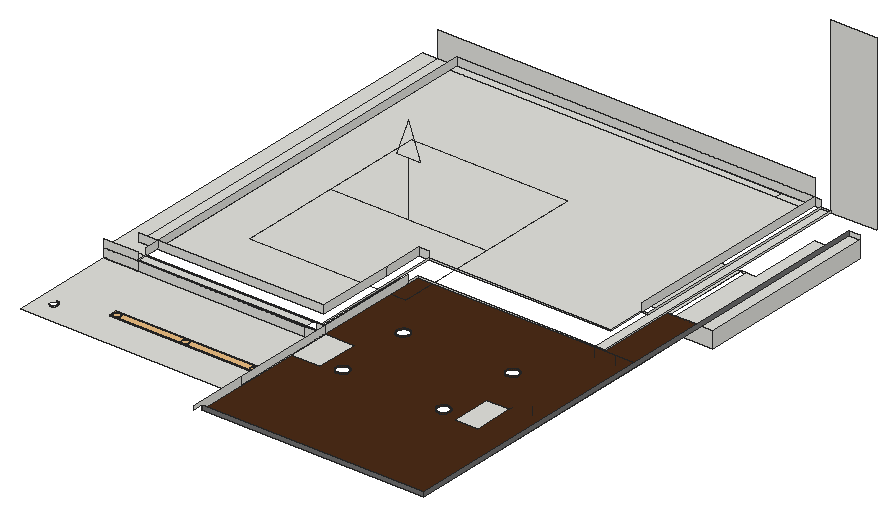
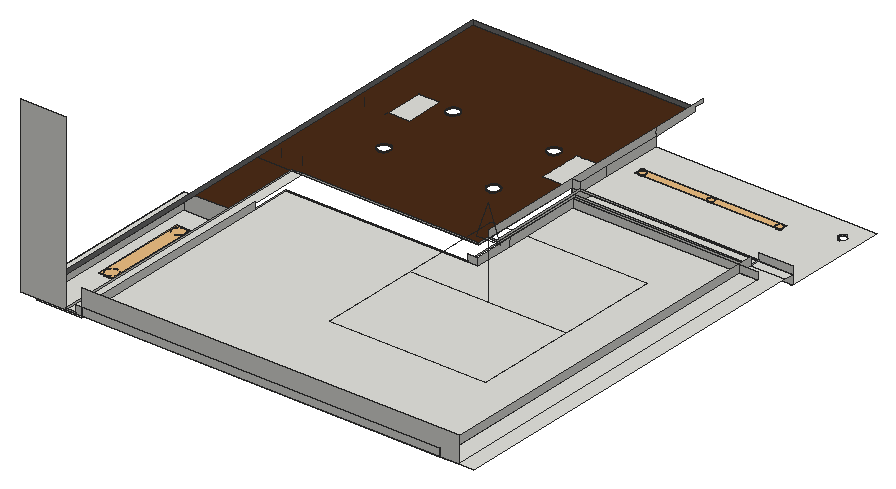
# SketchUp Ruby script. Lengths in inches.
U = 1.inch
M = Sketchup.active_model
def pt(a) = Geom::Point3d.new(a.map { |v| v * U })
def face(e, loops, mat)
  f = e.add_face(loops[0].map { |a| pt(a) })
  loops[1..].each { |l| e.add_face(l.map { |a| pt(a) }).erase! }
  f.material = f.back_material = mat if mat
  f
end
# faces: each face lists its corners as indices into pts; further lists are holes
def faces(e, pts, list, mat = nil) = list.each { |f| face(e, (f[0].is_a?(Array) ? f : [f]).map { |l| l.map { |i| pts[i] } }, mat) }
# xy, xz, yz: faces in a plane at the given z, y or x. An outline is a flat list of corners, or four numbers for a rectangle; further outlines are holes
def ring(l) = l.size == 4 ? [[l[0], l[1]], [l[2], l[1]], [l[2], l[3]], [l[0], l[3]]] : l.each_slice(2).to_a
def flat(e, list, mat, &to3) = list.each { |f| face(e, (f[0].is_a?(Array) ? f : [f]).map { |l| ring(l).map { |u, v| to3.(u, v) } }, mat) }
def xy(e, z, list, mat = nil) = flat(e, list, mat) { |x, y| [x, y, z] }
def xz(e, y, list, mat = nil) = flat(e, list, mat) { |x, z| [x, y, z] }
def yz(e, x, list, mat = nil) = flat(e, list, mat) { |y, z| [x, y, z] }
def lines(e, pts, list) = list.each { |a, b| e.add_line(pt(pts[a]), pt(pts[b])) }
# prism: a flat outline (further loops are holes) pulled along v
def prism(e, loops, v, mat = nil)
  f = face(e, loops, mat); d = Geom::Vector3d.new(v.map { |x| x * U })
  f.pushpull(f.normal.samedirection?(d) ? d.length : -d.length)
end
def box(e, o, s, mat = nil) = prism(e, [[o, [o[0] + s[0], o[1], o[2]], [o[0] + s[0], o[1] + s[1], o[2]], [o[0], o[1] + s[1], o[2]]]], [0, 0, s[2]], mat)
def at(x, y, z, deg = 0) = Geom::Transformation.translation(pt([x, y, z])) * Geom::Transformation.rotation(ORIGIN, Z_AXIS, deg.degrees)
def axes(o, x, y, z) = Geom::Transformation.new([*x, 0, *y, 0, *z, 0, *pt(o).to_a, 1])
def part(name) = M.definitions.add(name)
# library, detail: a bought-in or finely detailed component or shape, given as its bounding box
def library(name, o, s) = part(name).tap { |d| box(d.entities, o, s) }
def detail(e, o, s) = box(e.add_group.entities, o, s)
def put(e, d, t, mat = nil) = e.add_instance(d, t).tap { |i| i.material = mat if mat }
def group(e, t, mat = nil) = e.add_group.tap { |g| g.transformation = t; g.material = mat if mat }.entities
root = M.entities
M.materials.add("[Color M05]").color = [114, 114, 114]
M.materials.add("[Wood Veneer 01]").color = [76, 44, 23]
c1 = library("Group\#20",[-0.5,-0.5,-0.1],[139.5,7.875,0.2])
c2 = part("Group266\#1")
p = [[0,0,0],[0,0,-53.16],[-11.52,0,-53.16],[75.01,-97.09,0],[-75.01,-97.09,0],[75.01,97.09,0],
  [75.01,0,0],[-75.01,97.09,0],[11.52,0,-53.16],[-75.01,0,0],[0,0,-86.05]]
lines(c2.entities,p,[[0,1],[1,2],[3,4],[5,6],[7,5],[1,8],[9,0],[0,6],[8,10],[4,9],[6,3],[2,10],
  [9,7]])
c3 = part("Rectangle Light\#1")
put(c3.entities,c2,at(0,0,0))
c4 = library("Group\#22",[-0.5,-0.5,-0.1],[13.19,93.55,0.2])
xy(root,102.625,[[[3349.13,1821.9,3349.13,1844.2,3339.91,1844.2,3339.91,1928.83,3349.13,1928.83,3349.13,1998.71,3392.88,1998.71,3392.88,1821.9],[3374.07,1926.22,3375.65,1926.42,3377.12,1927.03,3378.38,1928,3379.35,1929.26,3379.96,1930.73,3380.16,1932.31,3379.96,1933.89,3379.35,1935.35,3378.38,1936.62,3377.12,1937.58,3375.65,1938.19,3374.07,1938.4,3372.49,1938.19,3371.02,1937.58,3369.76,1936.62,3368.79,1935.35,3368.1875,1933.89,3367.98,1932.31,3368.1875,1930.73,3368.79,1929.26,3369.76,1928,3371.02,1927.03,3372.49,1926.42],[3374.07,1845.85,3375.625,1846.05,3377.07,1846.65,3378.3125,1847.61,3379.27,1848.85,3379.87,1850.3,3380.07,1851.85,3379.87,1853.4,3379.27,1854.85,3378.3125,1856.09,3377.07,1857.05,3375.625,1857.65,3374.07,1857.85,3372.52,1857.65,3371.07,1857.05,3369.83,1856.09,3368.875,1854.85,3368.28,1853.4,3368.07,1851.85,3368.28,1850.3,3368.875,1848.85,3369.83,1847.61,3371.07,1846.65,3372.52,1846.05]],[3240.94,1844.2,3334.66,1928.14],[3334.66,1844.2,3335.34,1928.83],[3240.94,1928.14,3334.66,1928.83],[3335.34,1928.14,3336.03,1928.14,3336.03,1928.27,3339.91,1928.27,3339.91,1928.83,3335.34,1928.83],
  [3336.03,1928.14,3339.91,1928.27]])
xy(root,109.625,[[[2957.51,1535.54,3169.48,1636.04],[2972.07,1553.19,2973.125,1553.33,2974.1,1553.73,2974.95,1554.38,2975.59,1555.22,2976,1556.2,2976.14,1557.25,2976,1558.3,2975.59,1559.28,2974.95,1560.125,2974.1,1560.77,2973.125,1561.18,2972.07,1561.31,2971.02,1561.18,2970.04,1560.77,2969.2,1560.125,2968.55,1559.28,2968.15,1558.3,2968.01,1557.25,2968.15,1556.2,2968.55,1555.22,2969.2,1554.38,2970.04,1553.73,2971.02,1553.33],[3020.13,1569.87,3021.02,1569.99,3021.85,1570.33,3022.56,1570.875,3023.11,1571.59,3023.45,1572.42,3023.57,1573.31,3023.45,1574.2,3023.11,1575.02,3022.56,1575.74,3021.85,1576.28,3021.02,1576.625,3020.13,1576.74,3019.24,1576.625,3018.41,1576.28,3017.7,1575.74,3017.15,1575.02,3016.81,1574.2,3016.69,1573.31,3016.81,1572.42,3017.15,1571.59,3017.7,1570.875,3018.41,1570.33,3019.24,1569.99],[3085.94,1569.87,3086.83,1569.99,3087.66,1570.33,3088.37,1570.875,3088.92,1571.59,3089.26,1572.42,3089.38,1573.31,3089.26,1574.2,3088.92,1575.02,3088.37,1575.74,3087.66,1576.28,3086.83,1576.625,3085.94,1576.74,3085.05,1576.625,3084.22,1576.28,3083.51,1575.74,3082.96,1575.02,3082.62,1574.2,3082.5,1573.31,3082.62,1572.42,3082.96,1571.59,3083.51,1570.875,3084.22,1570.33,3085.05,1569.99],[3151.75,1569.87,3152.64,1569.99,3153.47,1570.33,3154.19,1570.875,3154.73,1571.59,3155.07,1572.42,3155.19,1573.31,3155.07,1574.2,3154.73,1575.02,3154.19,1575.74,3153.47,1576.28,3152.64,1576.625,3151.75,1576.74,3150.86,1576.625,3150.04,1576.28,3149.32,1575.74,3148.78,1575.02,3148.43,1574.2,3148.32,1573.31,3148.43,1572.42,3148.78,1571.59,3149.32,1570.875,3150.04,1570.33,3150.86,1569.99]]])
xy(root,118.5,[[3169.48,1595.04,3196.91,1635.98],[3327.63,1595.04,3349.13,1632.6],[2957.51,1636.04,2989.82,1645.27],[2989.82,1636.04,3150.65,1645.27],[2957.51,1645.27,2989.82,1645.27,2989.82,1659.57,2972.24,1659.57,2972.24,2018.36,2957.51,2018.36],
  [2972.24,1659.57,2989.82,2018.36],[2989.82,1659.57,2989.82,2010.98,3333.43,2010.98,3333.43,1773.67,3149.44,1773.67,3149.44,1659.57],[3339.91,1746.92,3349.13,2018.36],[3382.57,1821.9,3392.88,1998.71],[2989.82,2010.98,3302.57,2018.36],
  [3302.57,2010.98,3333.43,2018.36]])
xy(root,118.5,[[[3169.48,1488.17,3169.48,1595.04,3196.91,1595.04,3196.91,1635.98,3169.48,1635.98,3169.48,1746.92,3382.57,1746.92,3382.57,1488.17],[3327.63,1595.04,3349.13,1632.6],[3311.11,1595.24,3312.66,1595.44,3314.11,1596.04,3315.35,1596.99,3316.31,1598.24,3316.91,1599.68,3317.11,1601.24,3316.91,1602.79,3316.31,1604.24,3315.35,1605.48,3314.11,1606.43,3312.66,1607.03,3311.11,1607.24,3309.56,1607.03,3308.11,1606.43,3306.87,1605.48,3305.92,1604.24,3305.32,1602.79,3305.11,1601.24,3305.32,1599.68,3305.92,1598.24,3306.87,1596.99,3308.11,1596.04,3309.56,1595.44],[3214.3,1595.24,3215.85,1595.44,3217.3,1596.04,3218.54,1596.99,3219.5,1598.24,3220.09,1599.68,3220.3,1601.24,3220.09,1602.79,3219.5,1604.24,3218.54,1605.48,3217.3,1606.43,3215.85,1607.03,3214.3,1607.24,3212.75,1607.03,3211.3,1606.43,3210.06,1605.48,3209.1,1604.24,3208.5,1602.79,3208.3,1601.24,3208.5,1599.68,3209.1,1598.24,3210.06,1596.99,3211.3,1596.04,3212.75,1595.44],[3214.3,1667.99,3215.85,1668.19,3217.3,1668.79,3218.54,1669.74,3219.5,1670.99,3220.09,1672.43,3220.3,1673.99,3220.09,1675.54,3219.5,1676.99,3218.54,1678.23,3217.3,1679.18,3215.85,1679.78,3214.3,1679.99,3212.75,1679.78,3211.3,1679.18,3210.06,1678.23,3209.1,1676.99,3208.5,1675.54,3208.3,1673.99,3208.5,1672.43,3209.1,1670.99,3210.06,1669.74,3211.3,1668.79,3212.75,1668.19],[3316.66,1671.22,3318.21,1671.43,3319.66,1672.03,3320.9,1672.98,3321.86,1674.22,3322.46,1675.67,3322.66,1677.22,3322.46,1678.77,3321.86,1680.22,3320.9,1681.46,3319.66,1682.42,3318.21,1683.02,3316.66,1683.22,3315.11,1683.02,3313.66,1682.42,3312.42,1681.46,3311.46,1680.22,3310.87,1678.77,3310.66,1677.22,3310.87,1675.67,3311.46,1674.22,3312.42,1672.98,3313.66,1672.03,3315.11,1671.43]],[3349.13,1746.92,3382.57,1821.9]],"[Wood Veneer 01]")
xz(root,1488.17,[[3169.48,118.5,3382.57,122.875]],"[Color M05]")
xz(root,1636.04,[[2957.51,109.5,2989.82,109.625],[2957.51,109.625,2989.82,118.5],[2989.82,109.625,3150.65,118.5],[3150.65,109.625,3169.48,118.5],[2957.51,118.5,2989.82,126],
  [2989.82,118.5,3162.07,119.75],[3162.07,118.5,3169.48,126]])
xz(root,1645.27,[[2989.82,118.5,3159.13,119.75]])
xz(root,1659.57,[[2972.24,118.5,3149.44,126]])
xz(root,1735.1,[[3162.07,118.5,3169.48,119.75]])
xz(root,1746.92,[[3169.48,118.5,3339.91,119.75],[3339.91,118.5,3349.13,119.75]])
xz(root,1773.67,[[3149.44,118.5,3159.13,126],[3159.13,118.5,3333.43,119.75]])
xz(root,1810.9,[[3333.43,118.5,3339.91,119.75]])
xz(root,1821.9,[[3349.13,102.625,3392.88,118.5]])
xz(root,1998.71,[[3382.57,118.5,3392.88,122.875]])
xz(root,2018.36,[[2972.24,118.5,2972.24,142.875,3333.43,142.875,3333.43,126,2989.82,126,2989.82,118.5],[2989.82,118.5,3333.43,126],[3333.43,118.5,3339.91,126],[3339.91,118.5,3349.13,119.75],[3349.13,118.5,3392.88,283.9375]])
yz(root,2989.82,[[1636.04,118.5,1645.27,119.75],[1645.27,118.5,2018.36,126]])
yz(root,3149.44,[[1659.57,118.5,1735.1,126],[1735.1,118.5,1773.67,126]])
yz(root,3159.13,[[1645.27,118.5,1773.67,119.75]])
yz(root,3162.07,[[1636.04,118.5,1735.1,119.75]])
yz(root,3169.48,[[1535.54,109.625,1595.04,118.5],[1595.04,109.625,1635.98,118.5],[1635.98,109.625,1636.04,118.5],[1488.17,118.5,1488.17,122.875,1478.85,122.875,1478.85,126,1535.54,126,1535.54,118.5],[1535.54,118.5,1636.04,126],
  [1636.04,118.5,1735.1,126],[1735.1,118.5,1746.92,119.75]])
yz(root,3333.43,[[1773.67,118.5,1810.9,119.75],[1810.9,118.5,2018.36,126]])
yz(root,3339.91,[[1810.9,118.5,2018.36,119.75]])
yz(root,3349.13,[[1746.92,118.5,2018.36,119.75]])
yz(root,3382.57,[[1488.17,118.5,1998.71,122.875]],"[Color M05]")
yz(root,3392.88,[[1821.9,102.625,1998.71,118.5]])
p = [[3374.07,1845.85,102.625],[3372.52,1846.05,102.625],[3372.52,1846.05,103.9375],[3374.07,1845.85,103.9375],[3375.625,1846.05,102.625],[3375.625,1846.05,103.9375],
  [3371.07,1846.65,102.625],[3371.07,1846.65,103.9375],[3377.07,1846.65,102.625],[3377.07,1846.65,103.9375],[3369.83,1847.61,102.625],[3369.83,1847.61,103.9375],
  [3378.3125,1847.61,102.625],[3378.3125,1847.61,103.9375],[3368.875,1848.85,102.625],[3368.875,1848.85,103.9375],[3379.27,1848.85,102.625],[3379.27,1848.85,103.9375],
  [3368.28,1850.3,102.625],[3368.28,1850.3,103.9375],[3379.87,1850.3,102.625],[3379.87,1850.3,103.9375],[3368.07,1851.85,102.625],[3368.07,1851.85,103.9375],
  [3380.07,1851.85,102.625],[3380.07,1851.85,103.9375],[3368.28,1853.4,102.625],[3368.28,1853.4,103.9375],[3379.87,1853.4,102.625],[3379.87,1853.4,103.9375],
  [3368.875,1854.85,102.625],[3368.875,1854.85,103.9375],[3379.27,1854.85,102.625],[3379.27,1854.85,103.9375],[3369.83,1856.09,102.625],[3369.83,1856.09,103.9375],
  [3378.3125,1856.09,102.625],[3378.3125,1856.09,103.9375],[3371.07,1857.05,102.625],[3371.07,1857.05,103.9375],[3377.07,1857.05,102.625],[3377.07,1857.05,103.9375],
  [3372.52,1857.65,102.625],[3372.52,1857.65,103.9375],[3375.625,1857.65,102.625],[3375.625,1857.65,103.9375],[3374.07,1857.85,102.625],[3374.07,1857.85,103.9375],
  [3374.07,1926.22,102.625],[3372.49,1926.42,102.625],[3372.49,1926.42,103.9375],[3374.07,1926.22,103.9375],[3375.65,1926.42,102.625],[3375.65,1926.42,103.9375],
  [3371.02,1927.03,102.625],[3371.02,1927.03,103.9375],[3377.12,1927.03,102.625],[3377.12,1927.03,103.9375],[3369.76,1928,102.625],[3369.76,1928,103.9375],
  [3378.38,1928,102.625],[3378.38,1928,103.9375],[3368.79,1929.26,102.625],[3368.79,1929.26,103.9375],[3379.35,1929.26,102.625],[3379.35,1929.26,103.9375],
  [3368.1875,1930.73,102.625],[3368.1875,1930.73,103.9375],[3379.96,1930.73,102.625],[3379.96,1930.73,103.9375],[3367.98,1932.31,102.625],[3367.98,1932.31,103.9375],
  [3380.16,1932.31,102.625],[3380.16,1932.31,103.9375],[3368.1875,1933.89,102.625],[3368.1875,1933.89,103.9375],[3379.96,1933.89,102.625],[3379.96,1933.89,103.9375],
  [3368.79,1935.35,102.625],[3368.79,1935.35,103.9375],[3379.35,1935.35,102.625],[3379.35,1935.35,103.9375],[3369.76,1936.62,102.625],[3369.76,1936.62,103.9375],
  [3378.38,1936.62,102.625],[3378.38,1936.62,103.9375],[3371.02,1937.58,102.625],[3371.02,1937.58,103.9375],[3377.12,1937.58,102.625],[3377.12,1937.58,103.9375],
  [3372.49,1938.19,102.625],[3372.49,1938.19,103.9375],[3375.65,1938.19,102.625],[3375.65,1938.19,103.9375],[3374.07,1938.4,102.625],[3374.07,1938.4,103.9375],
  [2973.125,1553.33,109.625],[2972.07,1553.19,109.625],[2972.07,1553.19,110.5625],[2973.125,1553.33,110.5625],[2974.1,1553.73,109.625],[2974.1,1553.73,110.5625],
  [2974.95,1554.38,109.625],[2974.95,1554.38,110.5625],[2975.59,1555.22,109.625],[2975.59,1555.22,110.5625],[2976,1556.2,109.625],[2976,1556.2,110.5625],
  [2976.14,1557.25,109.625],[2976.14,1557.25,110.5625],[2976,1558.3,109.625],[2976,1558.3,110.5625],[2975.59,1559.28,109.625],[2975.59,1559.28,110.5625],
  [2974.95,1560.125,109.625],[2974.95,1560.125,110.5625],[2974.1,1560.77,109.625],[2974.1,1560.77,110.5625],[2973.125,1561.18,109.625],[2973.125,1561.18,110.5625],
  [2972.07,1561.31,109.625],[2972.07,1561.31,110.5625],[3020.13,1569.87,109.625],[3019.24,1569.99,109.625],[3019.24,1569.99,110.0625],[3020.13,1569.87,110.0625],
  [3021.02,1569.99,109.625],[3021.02,1569.99,110.0625],[3085.94,1569.87,109.625],[3085.05,1569.99,109.625],[3085.05,1569.99,110.0625],[3085.94,1569.87,110.0625],
  [3086.83,1569.99,109.625],[3086.83,1569.99,110.0625],[3151.75,1569.87,109.625],[3150.86,1569.99,109.625],[3150.86,1569.99,110.0625],[3151.75,1569.87,110.0625],
  [3152.64,1569.99,109.625],[3152.64,1569.99,110.0625],[3018.41,1570.33,109.625],[3018.41,1570.33,110.0625],[3021.85,1570.33,109.625],[3021.85,1570.33,110.0625],
  [3084.22,1570.33,109.625],[3084.22,1570.33,110.0625],[3087.66,1570.33,109.625],[3087.66,1570.33,110.0625],[3150.04,1570.33,109.625],[3150.04,1570.33,110.0625],
  [3153.47,1570.33,109.625],[3153.47,1570.33,110.0625],[3017.7,1570.875,109.625],[3017.7,1570.875,110.0625],[3022.56,1570.875,109.625],[3022.56,1570.875,110.0625],
  [3083.51,1570.875,109.625],[3083.51,1570.875,110.0625],[3088.37,1570.875,109.625],[3088.37,1570.875,110.0625],[3149.32,1570.875,109.625],[3149.32,1570.875,110.0625],
  [3154.19,1570.875,109.625],[3154.19,1570.875,110.0625],[3017.15,1571.59,109.625],[3017.15,1571.59,110.0625],[3023.11,1571.59,109.625],[3023.11,1571.59,110.0625],
  [3082.96,1571.59,109.625],[3082.96,1571.59,110.0625],[3088.92,1571.59,109.625],[3088.92,1571.59,110.0625],[3148.78,1571.59,109.625],[3148.78,1571.59,110.0625],
  [3154.73,1571.59,109.625],[3154.73,1571.59,110.0625],[3016.81,1572.42,109.625],[3016.81,1572.42,110.0625],[3023.45,1572.42,109.625],[3023.45,1572.42,110.0625],
  [3082.62,1572.42,109.625],[3082.62,1572.42,110.0625],[3089.26,1572.42,109.625],[3089.26,1572.42,110.0625],[3148.43,1572.42,109.625],[3148.43,1572.42,110.0625],
  [3155.07,1572.42,109.625],[3155.07,1572.42,110.0625],[3016.69,1573.31,109.625],[3016.69,1573.31,110.0625],[3023.57,1573.31,109.625],[3023.57,1573.31,110.0625],
  [3082.5,1573.31,109.625],[3082.5,1573.31,110.0625],[3089.38,1573.31,109.625],[3089.38,1573.31,110.0625],[3148.32,1573.31,109.625],[3148.32,1573.31,110.0625],
  [3155.19,1573.31,109.625],[3155.19,1573.31,110.0625],[3016.81,1574.2,109.625],[3016.81,1574.2,110.0625],[3023.45,1574.2,109.625],[3023.45,1574.2,110.0625],
  [3082.62,1574.2,109.625],[3082.62,1574.2,110.0625],[3089.26,1574.2,109.625],[3089.26,1574.2,110.0625],[3148.43,1574.2,109.625],[3148.43,1574.2,110.0625],
  [3155.07,1574.2,109.625],[3155.07,1574.2,110.0625],[3017.15,1575.02,109.625],[3017.15,1575.02,110.0625],[3023.11,1575.02,109.625],[3023.11,1575.02,110.0625],
  [3082.96,1575.02,109.625],[3082.96,1575.02,110.0625],[3088.92,1575.02,109.625],[3088.92,1575.02,110.0625],[3148.78,1575.02,109.625],[3148.78,1575.02,110.0625],
  [3154.73,1575.02,109.625],[3154.73,1575.02,110.0625],[3017.7,1575.74,109.625],[3017.7,1575.74,110.0625],[3022.56,1575.74,109.625],[3022.56,1575.74,110.0625],
  [3083.51,1575.74,109.625],[3083.51,1575.74,110.0625],[3088.37,1575.74,109.625],[3088.37,1575.74,110.0625],[3149.32,1575.74,109.625],[3149.32,1575.74,110.0625],
  [3154.19,1575.74,109.625],[3154.19,1575.74,110.0625],[3018.41,1576.28,109.625],[3018.41,1576.28,110.0625],[3021.85,1576.28,109.625],[3021.85,1576.28,110.0625],
  [3084.22,1576.28,109.625],[3084.22,1576.28,110.0625],[3087.66,1576.28,109.625],[3087.66,1576.28,110.0625],[3150.04,1576.28,109.625],[3150.04,1576.28,110.0625],
  [3153.47,1576.28,109.625],[3153.47,1576.28,110.0625],[3019.24,1576.625,109.625],[3019.24,1576.625,110.0625],[3021.02,1576.625,109.625],[3021.02,1576.625,110.0625],
  [3085.05,1576.625,109.625],[3085.05,1576.625,110.0625],[3086.83,1576.625,109.625],[3086.83,1576.625,110.0625],[3150.86,1576.625,109.625],[3150.86,1576.625,110.0625],
  [3152.64,1576.625,109.625],[3152.64,1576.625,110.0625],[3020.13,1576.74,109.625],[3020.13,1576.74,110.0625],[3085.94,1576.74,109.625],[3085.94,1576.74,110.0625],
  [3151.75,1576.74,109.625],[3151.75,1576.74,110.0625],[3214.3,1595.24,118.5],[3212.75,1595.44,118.5],[3212.75,1595.44,119.375],[3214.3,1595.24,119.375],
  [3215.85,1595.44,118.5],[3215.85,1595.44,119.375],[3311.11,1595.24,118.5],[3309.56,1595.44,118.5],[3309.56,1595.44,119.375],[3311.11,1595.24,119.375],
  [3312.66,1595.44,118.5],[3312.66,1595.44,119.375],[3211.3,1596.04,118.5],[3211.3,1596.04,119.375],[3217.3,1596.04,118.5],[3217.3,1596.04,119.375],
  [3308.11,1596.04,118.5],[3308.11,1596.04,119.375],[3314.11,1596.04,118.5],[3314.11,1596.04,119.375],[3210.06,1596.99,118.5],[3210.06,1596.99,119.375],
  [3218.54,1596.99,118.5],[3218.54,1596.99,119.375],[3306.87,1596.99,118.5],[3306.87,1596.99,119.375],[3315.35,1596.99,118.5],[3315.35,1596.99,119.375],
  [3209.1,1598.24,118.5],[3209.1,1598.24,119.375],[3219.5,1598.24,118.5],[3219.5,1598.24,119.375],[3305.92,1598.24,118.5],[3305.92,1598.24,119.375],
  [3316.31,1598.24,118.5],[3316.31,1598.24,119.375],[3208.5,1599.68,118.5],[3208.5,1599.68,119.375],[3220.09,1599.68,118.5],[3220.09,1599.68,119.375],
  [3305.32,1599.68,118.5],[3305.32,1599.68,119.375],[3316.91,1599.68,118.5],[3316.91,1599.68,119.375],[3208.3,1601.24,118.5],[3208.3,1601.24,119.375],
  [3220.3,1601.24,118.5],[3220.3,1601.24,119.375],[3305.11,1601.24,118.5],[3305.11,1601.24,119.375],[3317.11,1601.24,118.5],[3317.11,1601.24,119.375],
  [3208.5,1602.79,118.5],[3208.5,1602.79,119.375],[3220.09,1602.79,118.5],[3220.09,1602.79,119.375],[3305.32,1602.79,118.5],[3305.32,1602.79,119.375],
  [3316.91,1602.79,118.5],[3316.91,1602.79,119.375],[3209.1,1604.24,118.5],[3209.1,1604.24,119.375],[3219.5,1604.24,118.5],[3219.5,1604.24,119.375],
  [3305.92,1604.24,118.5],[3305.92,1604.24,119.375],[3316.31,1604.24,118.5],[3316.31,1604.24,119.375],[3210.06,1605.48,118.5],[3210.06,1605.48,119.375],
  [3218.54,1605.48,118.5],[3218.54,1605.48,119.375],[3306.87,1605.48,118.5],[3306.87,1605.48,119.375],[3315.35,1605.48,118.5],[3315.35,1605.48,119.375],
  [3211.3,1606.43,118.5],[3211.3,1606.43,119.375],[3217.3,1606.43,118.5],[3217.3,1606.43,119.375],[3308.11,1606.43,118.5],[3308.11,1606.43,119.375],
  [3314.11,1606.43,118.5],[3314.11,1606.43,119.375],[3212.75,1607.03,118.5],[3212.75,1607.03,119.375],[3215.85,1607.03,118.5],[3215.85,1607.03,119.375],
  [3309.56,1607.03,118.5],[3309.56,1607.03,119.375],[3312.66,1607.03,118.5],[3312.66,1607.03,119.375],[3214.3,1607.24,118.5],[3214.3,1607.24,119.375],
  [3311.11,1607.24,118.5],[3311.11,1607.24,119.375],[3214.3,1667.99,118.5],[3212.75,1668.19,118.5],[3212.75,1668.19,119.375],[3214.3,1667.99,119.375],
  [3215.85,1668.19,118.5],[3215.85,1668.19,119.375],[3211.3,1668.79,118.5],[3211.3,1668.79,119.375],[3217.3,1668.79,118.5],[3217.3,1668.79,119.375],
  [3210.06,1669.74,118.5],[3210.06,1669.74,119.375],[3218.54,1669.74,118.5],[3218.54,1669.74,119.375],[3209.1,1670.99,118.5],[3209.1,1670.99,119.375],
  [3219.5,1670.99,118.5],[3219.5,1670.99,119.375],[3208.5,1672.43,118.5],[3208.5,1672.43,119.375],[3220.09,1672.43,118.5],[3220.09,1672.43,119.375],
  [3316.66,1671.22,118.5],[3315.11,1671.43,118.5],[3315.11,1671.43,119.375],[3316.66,1671.22,119.375],[3318.21,1671.43,118.5],[3318.21,1671.43,119.375],
  [3313.66,1672.03,118.5],[3313.66,1672.03,119.375],[3319.66,1672.03,118.5],[3319.66,1672.03,119.375],[3312.42,1672.98,118.5],[3312.42,1672.98,119.375],
  [3320.9,1672.98,118.5],[3320.9,1672.98,119.375],[3208.3,1673.99,118.5],[3208.3,1673.99,119.375],[3220.3,1673.99,118.5],[3220.3,1673.99,119.375],
  [3311.46,1674.22,118.5],[3311.46,1674.22,119.375],[3321.86,1674.22,118.5],[3321.86,1674.22,119.375],[3208.5,1675.54,118.5],[3208.5,1675.54,119.375],
  [3220.09,1675.54,118.5],[3220.09,1675.54,119.375],[3310.87,1675.67,118.5],[3310.87,1675.67,119.375],[3322.46,1675.67,118.5],[3322.46,1675.67,119.375],
  [3209.1,1676.99,118.5],[3209.1,1676.99,119.375],[3219.5,1676.99,118.5],[3219.5,1676.99,119.375],[3310.66,1677.22,118.5],[3310.66,1677.22,119.375],
  [3322.66,1677.22,118.5],[3322.66,1677.22,119.375],[3210.06,1678.23,118.5],[3210.06,1678.23,119.375],[3218.54,1678.23,118.5],[3218.54,1678.23,119.375],
  [3310.87,1678.77,118.5],[3310.87,1678.77,119.375],[3322.46,1678.77,118.5],[3322.46,1678.77,119.375],[3211.3,1679.18,118.5],[3211.3,1679.18,119.375],
  [3217.3,1679.18,118.5],[3217.3,1679.18,119.375],[3311.46,1680.22,118.5],[3311.46,1680.22,119.375],[3321.86,1680.22,118.5],[3321.86,1680.22,119.375],
  [3212.75,1679.78,118.5],[3212.75,1679.78,119.375],[3215.85,1679.78,118.5],[3215.85,1679.78,119.375],[3214.3,1679.99,118.5],[3214.3,1679.99,119.375],
  [3312.42,1681.46,118.5],[3312.42,1681.46,119.375],[3320.9,1681.46,118.5],[3320.9,1681.46,119.375],[3313.66,1682.42,118.5],[3313.66,1682.42,119.375],
  [3319.66,1682.42,118.5],[3319.66,1682.42,119.375],[3315.11,1683.02,118.5],[3315.11,1683.02,119.375],[3318.21,1683.02,118.5],[3318.21,1683.02,119.375],
  [3316.66,1683.22,118.5],[3316.66,1683.22,119.375],[3349.13,1735.1,126],[3349.13,1735.1,118.5],[3368.57,1735.1,126],[3368.57,1735.1,118.5],
  [3368.57,1636.04,118.5],[3368.57,1635.98,118.5],[3349.13,1635.98,118.5],[3349.13,1632.6,118.5],[3368.57,1636.04,126]]
faces(root,p,[[0,1,2,3],[4,0,3,5],[1,6,7,2],[8,4,5,9],[6,10,11,7],[12,8,9,13],[10,14,15,11],[16,12,13,17],
  [14,18,19,15],[20,16,17,21],[18,22,23,19],[24,20,21,25],[22,26,27,23],[28,24,25,29],[26,30,31,27],[32,28,29,33],
  [30,34,35,31],[36,32,33,37],[34,38,39,35],[40,36,37,41],[38,42,43,39],[44,40,41,45],[42,46,47,43],[46,44,45,47],
  [48,49,50,51],[52,48,51,53],[49,54,55,50],[56,52,53,57],[54,58,59,55],[60,56,57,61],[58,62,63,59],[64,60,61,65],
  [62,66,67,63],[68,64,65,69],[66,70,71,67],[72,68,69,73],[70,74,75,71],[76,72,73,77],[74,78,79,75],[80,76,77,81],
  [78,82,83,79],[84,80,81,85],[82,86,87,83],[88,84,85,89],[86,90,91,87],[92,88,89,93],[90,94,95,91],[94,92,93,95],
  [96,97,98,99],[100,96,99,101],[102,100,101,103],[104,102,103,105],[106,104,105,107],[108,106,107,109],[110,108,109,111],[112,110,111,113],
  [114,112,113,115],[116,114,115,117],[118,116,117,119],[120,118,119,121],[122,123,124,125],[126,122,125,127],[128,129,130,131],[132,128,131,133],
  [134,135,136,137],[138,134,137,139],[123,140,141,124],[142,126,127,143],[129,144,145,130],[146,132,133,147],[135,148,149,136],[150,138,139,151],
  [140,152,153,141],[154,142,143,155],[144,156,157,145],[158,146,147,159],[148,160,161,149],[162,150,151,163],[152,164,165,153],[166,154,155,167],
  [156,168,169,157],[170,158,159,171],[160,172,173,161],[174,162,163,175],[164,176,177,165],[178,166,167,179],[168,180,181,169],[182,170,171,183],
  [172,184,185,173],[186,174,175,187],[176,188,189,177],[190,178,179,191],[180,192,193,181],[194,182,183,195],[184,196,197,185],[198,186,187,199],
  [188,200,201,189],[202,190,191,203],[192,204,205,193],[206,194,195,207],[196,208,209,197],[210,198,199,211],[200,212,213,201],[214,202,203,215],
  [204,216,217,205],[218,206,207,219],[208,220,221,209],[222,210,211,223],[212,224,225,213],[226,214,215,227],[216,228,229,217],[230,218,219,231],
  [220,232,233,221],[234,222,223,235],[224,236,237,225],[238,226,227,239],[228,240,241,229],[242,230,231,243],[232,244,245,233],[246,234,235,247],
  [236,248,249,237],[250,238,239,251],[240,252,253,241],[254,242,243,255],[244,256,257,245],[258,246,247,259],[248,260,261,249],[260,250,251,261],
  [252,262,263,253],[262,254,255,263],[256,264,265,257],[264,258,259,265]])
faces(root,p,[[266,267,268,269],[270,266,269,271],[272,273,274,275],[276,272,275,277],[267,278,279,268],[280,270,271,281],[273,282,283,274],[284,276,277,285],
  [278,286,287,279],[288,280,281,289],[282,290,291,283],[292,284,285,293],[286,294,295,287],[296,288,289,297],[290,298,299,291],[300,292,293,301],
  [294,302,303,295],[304,296,297,305],[298,306,307,299],[308,300,301,309],[302,310,311,303],[312,304,305,313],[306,314,315,307],[316,308,309,317],
  [310,318,319,311],[320,312,313,321],[314,322,323,315],[324,316,317,325],[318,326,327,319],[328,320,321,329],[322,330,331,323],[332,324,325,333],
  [326,334,335,327],[336,328,329,337],[330,338,339,331],[340,332,333,341],[334,342,343,335],[344,336,337,345],[338,346,347,339],[348,340,341,349],
  [342,350,351,343],[352,344,345,353],[346,354,355,347],[356,348,349,357],[350,358,359,351],[358,352,353,359],[354,360,361,355],[360,356,357,361],
  [362,363,364,365],[366,362,365,367],[363,368,369,364],[370,366,367,371],[368,372,373,369],[374,370,371,375],[372,376,377,373],[378,374,375,379],
  [376,380,381,377],[382,378,379,383],[384,385,386,387],[388,384,387,389],[385,390,391,386],[392,388,389,393],[390,394,395,391],[396,392,393,397],
  [380,398,399,381],[400,382,383,401],[394,402,403,395],[404,396,397,405],[398,406,407,399],[408,400,401,409],[402,410,411,403],[412,404,405,413],
  [406,414,415,407],[416,408,409,417],[410,418,419,411],[420,412,413,421],[414,422,423,415],[424,416,417,425],[418,426,427,419],[428,420,421,429],
  [422,430,431,423],[432,424,425,433],[426,434,435,427],[436,428,429,437],[430,438,439,431],[440,432,433,441],[438,442,443,439],[442,440,441,443],
  [434,444,445,435],[446,436,437,447],[444,448,449,445],[450,446,447,451],[448,452,453,449],[454,450,451,455],[452,456,457,453],[456,454,455,457]],"[Wood Veneer 01]")
lines(root,p,[[458,459],[460,461],[462,463],[464,465],[462,466]])
put(root,c1,at(3016.69,1569.87,110.0625))
put(root,c3,axes([3109.1,1811.78,118.51],[1,0,0],[0,1,0],[0,0,-1]))
put(root,c4,at(3367.98,1845.85,103.9375))
